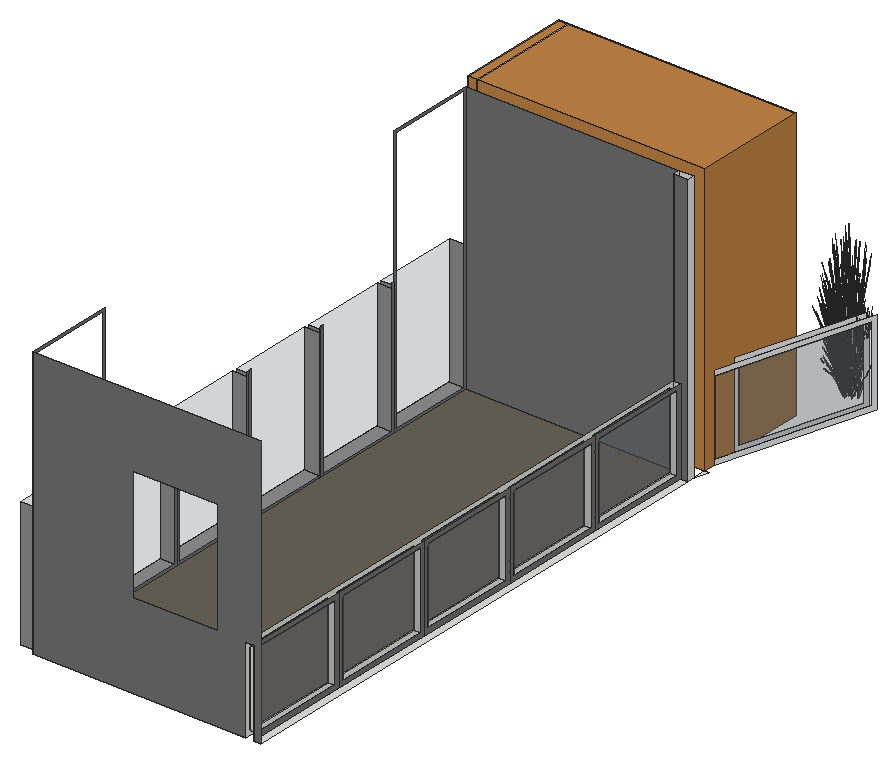
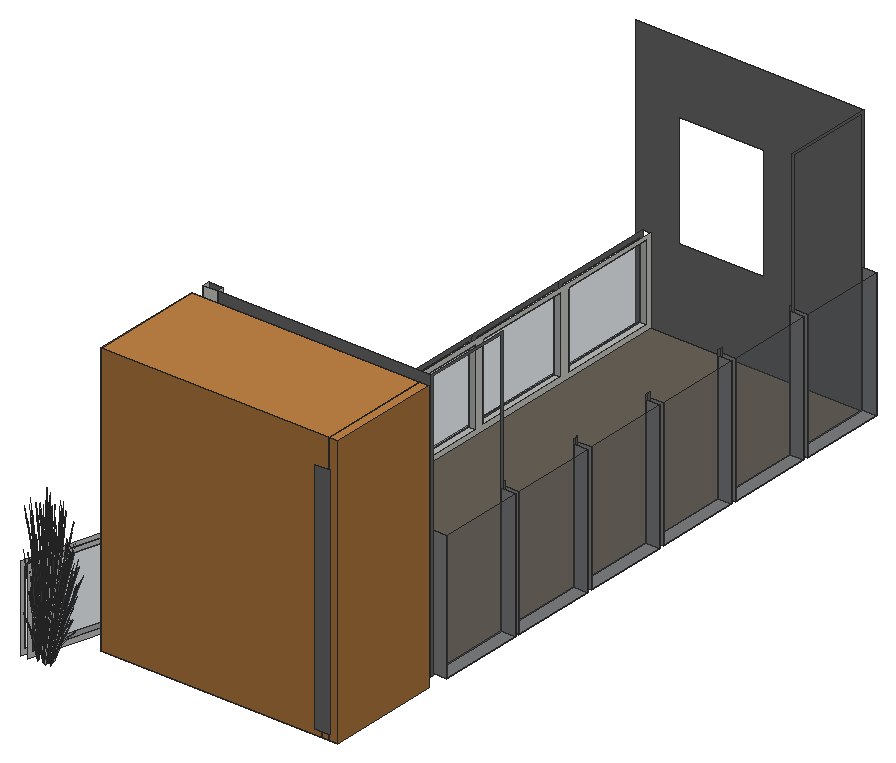
# SketchUp Ruby script. Lengths in inches.
U = 1.inch
M = Sketchup.active_model
def pt(a) = Geom::Point3d.new(a.map { |v| v * U })
def face(e, loops, mat)
  f = e.add_face(loops[0].map { |a| pt(a) })
  loops[1..].each { |l| e.add_face(l.map { |a| pt(a) }).erase! }
  f.material = f.back_material = mat if mat
  f
end
# faces: each face lists its corners as indices into pts; further lists are holes
def faces(e, pts, list, mat = nil) = list.each { |f| face(e, (f[0].is_a?(Array) ? f : [f]).map { |l| l.map { |i| pts[i] } }, mat) }
# xy, xz, yz: faces in a plane at the given z, y or x. An outline is a flat list of corners, or four numbers for a rectangle; further outlines are holes
def ring(l) = l.size == 4 ? [[l[0], l[1]], [l[2], l[1]], [l[2], l[3]], [l[0], l[3]]] : l.each_slice(2).to_a
def flat(e, list, mat, &to3) = list.each { |f| face(e, (f[0].is_a?(Array) ? f : [f]).map { |l| ring(l).map { |u, v| to3.(u, v) } }, mat) }
def xy(e, z, list, mat = nil) = flat(e, list, mat) { |x, y| [x, y, z] }
def xz(e, y, list, mat = nil) = flat(e, list, mat) { |x, z| [x, y, z] }
def yz(e, x, list, mat = nil) = flat(e, list, mat) { |y, z| [x, y, z] }
def lines(e, pts, list) = list.each { |a, b| e.add_line(pt(pts[a]), pt(pts[b])) }
# prism: a flat outline (further loops are holes) pulled along v
def prism(e, loops, v, mat = nil)
  f = face(e, loops, mat); d = Geom::Vector3d.new(v.map { |x| x * U })
  f.pushpull(f.normal.samedirection?(d) ? d.length : -d.length)
end
def box(e, o, s, mat = nil) = prism(e, [[o, [o[0] + s[0], o[1], o[2]], [o[0] + s[0], o[1] + s[1], o[2]], [o[0], o[1] + s[1], o[2]]]], [0, 0, s[2]], mat)
def at(x, y, z, deg = 0) = Geom::Transformation.translation(pt([x, y, z])) * Geom::Transformation.rotation(ORIGIN, Z_AXIS, deg.degrees)
def axes(o, x, y, z) = Geom::Transformation.new([*x, 0, *y, 0, *z, 0, *pt(o).to_a, 1])
def part(name) = M.definitions.add(name)
# library, detail: a bought-in or finely detailed component or shape, given as its bounding box
def library(name, o, s) = part(name).tap { |d| box(d.entities, o, s) }
def detail(e, o, s) = box(e.add_group.entities, o, s)
def put(e, d, t, mat = nil) = e.add_instance(d, t).tap { |i| i.material = mat if mat }
def group(e, t, mat = nil) = e.add_group.tap { |g| g.transformation = t; g.material = mat if mat }.entities
root = M.entities
M.materials.add("Glass_Basic_01").color = [105, 113, 122]
M.materials["Glass_Basic_01"].alpha = 0.25
M.materials.add("LightPink_Translucent").color = [144, 107, 117]
M.materials["LightPink_Translucent"].alpha = 0.75
M.materials.add("M01_Silver_Fog").color = [224, 224, 224]
M.materials.add("M04_Stone_Frost").color = [142, 142, 142]
M.materials.add("M06_Steel_Smoke").color = [114, 114, 114]
M.materials.add("Plaster_04_1K").color = [106, 98, 87]
M.materials.add("Wood_Floor_01_1K").color = [193, 132, 69]
c1 = part("Group\#1")
box(c1.entities,[-3.94,0,0],[99.94,48,114])
c2 = part("blade")
p = [[2.15,0.21,22],[0,0.17,0],[0.09,0.45,0],[2.18,0.31,22],[2.29,0.31,22],[0.38,0.45,0],
  [2.48,0.24,33],[2.49,0.24,33],[2.48,0.22,33]]
faces(c2.entities,p,[[0,1,2,3],[4,5,2,3],[6,3,4,7],[8,0,3,6]])
c3 = part("seeds")
p = [[0.3,-0.1,1.38],[-0.01,-0.03,1.59],[-0.01,-0.03,0.03],[0.14,-0.07,-0.07],[0.29,-0.03,3],[0.15,0.01,3.11]]
faces(c3.entities,p,[[0,1,2,3],[1,0,4,5]],"LightPink_Translucent")
c4 = part("blade with seeds")
put(c4.entities,c2,at(0,0,0))
put(c4.entities,c3,axes([2.4,0.25,30.99],[1.5799,-0.05474,1.17369],[-0.12525,1.92788,0.29478],[-0.07173,-0.02425,1.56792]))
xy(root,270,[[303,6,306,231],[306,234,307.76,240,306,240]])
xy(root,270,[[210,6,300,234]],"Plaster_04_1K")
xy(root,271,[[204,7,210,43],[204,45,210,81],[204,83,210,119],[204,121,210,157],[204,159,210,195],
  [204,197,210,233]],"M04_Stone_Frost")
xy(root,272,[[300,8,303,49],[300,53,303,94],[300,98,303,139],[300,143,303,184],[300,188,303,229]])
xz(root,6,[[[210,270,210,384,306,384,306,270,303,270,303,306,300,306,300,270],[252,306,288,354]]],"M06_Steel_Smoke")
xz(root,7,[[204,271,210,325]],"M04_Stone_Frost")
xz(root,8,[[300,272,303,304]])
xz(root,43,[[204,271,210,325]],"M04_Stone_Frost")
xz(root,45,[[204,271,210,325]],"M04_Stone_Frost")
xz(root,49,[[300,272,303,304]])
xz(root,53,[[300,272,303,304]])
xz(root,81,[[204,271,210,325]],"M04_Stone_Frost")
xz(root,83,[[204,271,210,325]],"M04_Stone_Frost")
xz(root,94,[[300,272,303,304]])
xz(root,98,[[300,272,303,304]])
xz(root,119,[[204,271,210,325]],"M04_Stone_Frost")
xz(root,121,[[204,271,210,325]],"M04_Stone_Frost")
xz(root,139,[[300,272,303,304]])
xz(root,143,[[300,272,303,304]])
xz(root,157,[[204,271,210,325]],"M04_Stone_Frost")
xz(root,159,[[204,271,210,325]],"M04_Stone_Frost")
xz(root,184,[[300,272,303,304]])
xz(root,188,[[300,272,303,304]])
xz(root,195,[[204,271,210,325]],"M04_Stone_Frost")
xz(root,197,[[204,271,210,325]],"M04_Stone_Frost")
xz(root,229,[[300,272,303,304]])
xz(root,231,[[303,270,306,270,306,384,300,384,300,306,303,306]],"M06_Steel_Smoke")
xz(root,233,[[204,271,210,325]],"M04_Stone_Frost")
xz(root,234,[[300,270,306,384]])
xz(root,234,[[210,270,300,384]],"M06_Steel_Smoke")
xz(root,243,[[213,270,305.51,306]],"M01_Silver_Fog")
xz(root,246,[[216,270,303.26,306]],"M01_Silver_Fog")
xz(root,287.79,[[213,270,216,306]],"M01_Silver_Fog")
xz(root,295,[[204,277,210,377]],"M06_Steel_Smoke")
yz(root,204,[[7,271,43,325],[45,271,81,325],[83,271,119,325],[121,271,157,325],[159,271,195,325],
  [197,271,233,325]],"Glass_Basic_01")
yz(root,210,[[240,270,288,270,288,316.46,286.46,316.46,286.46,337.54,288,337.54,288,384,240,384]])
yz(root,210,[[6,270,44,270,44,327,43,327,43,271,7,271,7,383,43,383,43,327,44,327,44,384,6,384],[44,270,82,270,82,327,81,327,81,271,45,271,45,327,44,327],[82,270,120,270,120,327,119,327,119,271,83,271,83,327,82,327],[120,270,158,270,158,327,157,327,157,271,121,271,121,327,120,327],[158,270,196,270,196,327,195,327,195,271,159,271,159,327,158,327],
  [196,270,234,270,234,384,196,384,196,327,197,327,197,383,233,383,233,271,197,271,197,327,196,327]],"M06_Steel_Smoke")
yz(root,213,[[243,270,287.79,306]],"M01_Silver_Fog")
yz(root,216,[[246,270,287.79,306]],"M01_Silver_Fog")
yz(root,300,[[[6,270,231,306],[8,272,49,304],[143,272,184,304],[188,272,229,304],[53,272,94,304],[98,272,139,304]],[231,270,234,384]])
yz(root,300,[[8,272,49,304],[53,272,94,304],[98,272,139,304],[143,272,184,304],[188,272,229,304]],"Glass_Basic_01")
yz(root,303,[[8,272,49,304],[53,272,94,304],[98,272,139,304],[143,272,184,304],[188,272,229,304]],"Glass_Basic_01")
yz(root,303,[[[6,270,51,306],[8,272,49,304]],[[51,270,96,306],[53,272,94,304]],[[96,270,141,306],[98,272,139,304]],[[141,270,186,306],[143,272,184,304]],[[186,270,231,306],[188,272,229,304]]],"M06_Steel_Smoke")
yz(root,306,[[231,270,234,384]])
p = [[305.51,243,270],[324.34,307.35,270],[324.34,307.35,306],[305.51,243,306],[323.78,305.43,304],[323.78,305.43,272],
  [306.07,244.92,272],[306.07,244.92,304],[303.26,246,306],[306,255.36,306],[306,255.36,270],[303.26,246,270],
  [321.22,307.35,306],[321.22,307.35,270],[320.65,305.43,304],[306.5625,257.28,304],[306.5625,257.28,272],[320.65,305.43,272],
  [209.78,288,384],[209.78,288,270],[305.48,242.91,270],[305.48,242.91,306]]
faces(root,p,[[[0,1,2,3],[4,5,6,7]],[8,9,10,11],[[9,12,13,10],[14,15,16,17]]],"M01_Silver_Fog")
faces(root,p,[[5,4,7,6],[15,14,17,16]],"Glass_Basic_01")
lines(root,p,[[18,19],[20,21]])
put(root,c1,at(210,240,270),"Wood_Floor_01_1K")
put(root,c4,axes([312.0625,305.99,273.875],[0.11485,0.17291,1.71376],[-0.53072,0.14557,0.13857],[-0.11995,-0.27145,0.73262]))
put(root,c4,axes([312.9375,304.84,274.72],[-0.07685,-0.07551,1.74944],[-0.51287,0.04787,-0.27667],[-0.08185,-0.1806,0.14031]))
put(root,c4,axes([314.125,305.74,272.59],[-0.14282,0.10901,1.43002],[-0.42773,-0.19079,-0.30754],[0.07929,-0.23728,0.61141]))
put(root,c4,axes([313.48,306.12,274.98],[-0.23981,-0.43789,-0.71045],[0.49365,-0.24404,0.08574],[-0.05608,-0.21158,1.00501]))
put(root,c4,axes([311.92,305.53,272.59],[-0.03043,0.17617,1.43002],[-0.4448,0.14748,-0.30754],[-0.10397,-0.22771,0.61141]))
put(root,c4,axes([313.0625,305.15,271.49],[-0.08428,0.0194,1.76342],[-0.46606,-0.21841,-0.26939],[0.00782,-0.18218,0.30037]))
put(root,c4,axes([314.47,306.55,274.98],[0.01307,-0.49815,-0.71045],[0.55054,0.03346,0.08574],[0.0581,-0.21104,1.00501]))
put(root,c4,axes([315.24,305.77,274.72],[-0.00485,-0.10718,1.74944],[-0.40965,-0.30977,-0.27667],[0.06333,-0.18778,0.14031]))
put(root,c4,axes([313.52,305.75,274.53],[0.15148,-0.41415,-0.35414],[0.44193,0.12079,0.4572],[-0.04052,-0.16674,0.87481]))
put(root,c4,axes([313.85,306.29,273.875],[-0.09355,0.18511,1.71376],[-0.39247,-0.38307,0.13857],[0.17705,-0.23875,0.73262]))
put(root,c4,axes([315.13,305.38,274.71],[-0.05103,0.04113,1.77383],[-0.49994,-0.13878,-0.16761],[-0.0181,-0.17951,0.31391]))
put(root,c4,axes([313.3,306.03,274.68],[-0.49392,-0.135,-0.51099],[0.1693,-0.46287,-0.3958],[-0.04529,-0.18636,0.97773]))
put(root,c4,axes([313.6,304.87,272.77],[0.06446,0.31404,1.1486],[-0.35756,-0.17393,0.84392],[0.03848,-0.1608,0.25299]))
put(root,c4,axes([314.36,306.38,274.68],[-0.35968,-0.36185,-0.51099],[0.37996,-0.3169,-0.3958],[0.05473,-0.18385,0.97773]))
put(root,c4,axes([312.41,304.6,274.71],[-0.00937,0.06455,1.77383],[-0.46231,0.23427,-0.16761],[-0.13604,-0.11975,0.31391]))
put(root,c4,axes([312.31,305.74,275.09],[0.55971,-0.13842,0.53763],[0.09714,0.54299,0.4433],[-0.13164,-0.16003,1.11249]))
put(root,c4,axes([313.58,305.84,274.73],[0.4951,0.14079,0.48003],[-0.1693,0.46287,0.3958],[-0.02975,-0.18203,0.9933]))
put(root,c4,axes([313.72,306.01,275.03],[-0.49168,0.25073,-0.1216],[-0.24162,-0.44501,-0.67495],[-0.06487,-0.18753,1.02557]))
put(root,c4,axes([314.74,306.57,275.03],[-0.55221,-0.02668,-0.1216],[0.01509,-0.50521,-0.67495],[0.03836,-0.19458,1.02557]))
put(root,c4,axes([314.7,306.25,274.53],[0.33997,-0.28354,-0.35414],[0.32182,0.32376,0.4572],[0.04897,-0.1645,0.87481]))
put(root,c4,axes([311.76,305.25,272.77],[0.2621,0.18744,1.1486],[-0.38171,0.11267,0.84392],[-0.08167,-0.14405,0.25299]))
put(root,c4,axes([313.71,305.81,274.73],[0.37023,-0.18303,0.0643],[0.18122,0.33376,0.50621],[-0.03575,-0.14712,0.77189]))
put(root,c4,axes([312.4,306.24,274.98],[-0.42844,-0.2603,-0.71045],[0.30448,-0.45614,0.08574],[-0.15523,-0.15542,1.00501]))
put(root,c4,axes([312.25,305.9,274.53],[-0.0776,-0.43378,-0.35414],[0.44361,-0.11454,0.4572],[-0.11915,-0.12431,0.87481]))
put(root,c4,axes([312.4375,305.86,274.73],[0.22836,-0.34211,0.0643],[0.3252,0.19918,0.50621],[-0.10513,-0.10968,0.77189]))
put(root,c4,axes([311.56,305.81,271.49],[-0.04867,0.07094,1.76342],[-0.49185,0.15296,-0.26939],[-0.11882,-0.13915,0.30037]))
put(root,c4,axes([312.37,307.76,272.1],[-0.20635,-0.55225,-0.69835],[0.59439,-0.19889,-0.18329],[-0.02281,-0.18701,1.54149]))
put(root,c4,axes([311.29,306.53,273.875],[0.18664,0.09279,1.71376],[-0.38624,0.38925,0.13857],[-0.24072,-0.1756,0.73262]))
put(root,c4,axes([315.125,306.08,271.49],[-0.0752,-0.04243,1.76342],[-0.19317,-0.47398,-0.26939],[0.13031,-0.12863,0.30037]))
put(root,c4,axes([313.57,306.18,275.05],[-0.15148,0.41415,0.35414],[-0.44193,-0.12079,-0.4572],[-0.04052,-0.16674,0.87481]))
put(root,c4,axes([312.19,306.26,274.68],[-0.4958,0.12802,-0.51099],[-0.08673,-0.48481,-0.3958],[-0.13317,-0.13893,0.97773]))
put(root,c4,axes([314.7,306.36,274.73],[0.35779,0.36745,0.48003],[-0.37996,0.3169,0.3958],[0.066,-0.17239,0.9933]))
put(root,c4,axes([312.54,305.82,275.43],[-0.33533,0.51628,-0.13619],[-0.48563,-0.29744,-0.75594],[-0.16881,-0.14586,1.14864]))
put(root,c4,axes([314.83,306.39,274.73],[0.4129,0.02509,0.0643],[-0.01132,0.37891,0.50621],[0.04321,-0.14514,0.77189]))
put(root,c4,axes([314.52,306.65,275.05],[-0.33997,0.28354,0.35414],[-0.32182,-0.32376,-0.4572],[0.04897,-0.1645,0.87481]))
put(root,c4,axes([315.12,307.41,274.98],[0.26246,-0.42493,-0.71045],[0.45991,0.30199,0.08574],[0.15671,-0.15395,1.00501]))
put(root,c4,axes([312.29,306.18,272.375],[-0.31414,-0.53965,0],[0.52557,-0.30095,-0.51607],[0.1197,-0.06854,1.63711]))
put(root,c4,axes([315.11,307.21,274.68],[-0.12908,-0.49174,-0.51099],[0.48882,-0.08602,-0.3958],[0.14008,-0.13208,0.97773]))
put(root,c4,axes([312.98,305.53,272.13],[-0.34721,0.30895,-0.03893],[-0.31814,-0.33837,-0.17649],[-0.0224,-0.09588,0.58215]))
put(root,c4,axes([311.26,305.67,274.72],[-0.10811,-0.0038,1.74944],[-0.34418,0.38014,-0.27667],[-0.18364,-0.07767,0.14031]))
put(root,c4,axes([315.34,307.57,275.03],[-0.46478,-0.29695,-0.1216],[0.26776,-0.43004,-0.67495],[0.13131,-0.14949,1.02557]))
put(root,c4,axes([313.42,309.1875,273.33],[0.4342,0.21716,1.51261],[-0.42537,0.46784,0.59816],[-0.19053,-0.27728,1.26806]))
put(root,c4,axes([312.51,306.25,275.05],[0.0776,0.43378,0.35414],[-0.44361,0.11454,-0.4572],[-0.11915,-0.12431,0.87481]))
put(root,c4,axes([311.15,307.6875,272.02],[0,-0.53854,-0.49651],[0.56215,0,0],[0,-0.12266,1.57504]))
put(root,c4,axes([312.71,306.09,272.02],[0.47024,-0.26927,-0.49651],[0.28107,0.48284,0],[0.1071,-0.06133,1.57504]))
put(root,c4,axes([315.5,307.02,272.59],[-0.1795,-0.01595,1.43002],[-0.18389,-0.42791,-0.30754],[0.22051,-0.12105,0.61141]))
put(root,c4,axes([311.18,306.53,275.09],[0.41494,-0.39744,0.53763],[0.35786,0.42207,0.4433],[-0.19468,-0.07331,1.11249]))
put(root,c4,axes([316.48,307.4375,274.71],[-0.06563,-0.00409,1.77383],[-0.27252,-0.43825,-0.16761],[0.10944,-0.1441,0.31391]))
put(root,c4,axes([313.27,307.2,272.06],[0.33843,-0.40479,-0.62353],[0.42041,0.36705,-0.16365],[0.13561,-0.10098,1.37633]))
put(root,c4,axes([315.71,306.24,272.77],[-0.16736,0.27414,1.1486],[-0.14385,-0.36832,0.84392],[0.13822,-0.09229,0.25299]))
put(root,c4,axes([315.47,307.27,274.53],[0.43736,-0.07697,-0.35414],[0.11549,0.43998,0.4572],[0.12533,-0.11818,0.87481]))
put(root,c4,axes([311.37,306.53,274.73],[0.0253,-0.40952,0.0643],[0.38204,0.01123,0.50621],[-0.14634,-0.04285,0.77189]))
put(root,c4,axes([312.68,307.91,272.21],[0.24378,-0.48527,-0.44739],[0.50654,0.23354,0.21531],[0,-0.11186,1.43643]))
put(root,c4,axes([311.22,306.66,274.53],[-0.28589,-0.33718,-0.35414],[0.32644,-0.31919,0.4572],[-0.16586,-0.04856,0.87481]))
put(root,c4,axes([312.9,307.67,272.67],[-0.05855,-0.61451,-0.29095],[0.60981,-0.03716,-0.50002],[0.10738,-0.08185,1.59708]))
put(root,c4,axes([311.39,307.7,272.03],[0.35073,-0.33601,-0.30978],[0.35073,0.33601,0.30978],[0,-0.10823,1.38974]))
put(root,c4,axes([311.25,306.09,272.13],[-0.14494,0.43975,-0.03893],[-0.4461,-0.13527,-0.17649],[-0.06773,-0.07192,0.58215]))
put(root,c4,axes([315.11,307.53,275.05],[-0.43736,0.07697,0.35414],[-0.11549,-0.43998,-0.4572],[0.12533,-0.11818,0.87481]))
put(root,c4,axes([312.62,308.31,272.67],[-0.56585,-0.25696,-0.29095],[0.27246,-0.54236,-0.50002],[-0.01778,-0.13316,1.59708]))
put(root,c4,axes([311.01,308.1,272.375],[-0.62828,0,0],[0,-0.6019,-0.51607],[0,-0.13709,1.63711]))
put(root,c4,axes([311.12,307.02,272.59],[0.0981,0.14994,1.43002],[-0.22605,0.40756,-0.30754],[-0.23211,-0.09741,0.61141]))
put(root,c4,axes([312.82,306.31,272.03],[0.46876,0.13325,-0.30978],[-0.11803,0.46926,0.30978],[0.0945,-0.05411,1.38974]))
put(root,c4,axes([311.52,306.89,274.98],[-0.50227,-0.01297,-0.71045],[0.03373,-0.54602,0.08574],[-0.21278,-0.05762,1.00501]))
put(root,c4,axes([315.51,307.46,274.73],[0.34493,0.22649,0.0643],[-0.20082,0.32253,0.50621],[0.11059,-0.10427,0.77189]))
put(root,c4,axes([315.41,307.36,274.73],[0.12461,0.49565,0.48003],[-0.48882,0.08602,0.3958],[0.14406,-0.11657,0.9933]))
put(root,c4,axes([316.73,307.96,274.72],[0.06972,-0.08203,1.74944],[-0.08924,-0.50318,-0.27667],[0.17494,-0.0954,0.14031]))
put(root,c4,axes([311.5,307.9375,272.33],[-0.46736,0.45277,0.30756],[-0.46764,-0.44801,-0.36492],[-0.01632,-0.12858,1.64885]))
put(root,c4,axes([310.84,306,274.71],[0.03725,0.05374,1.77383],[-0.17957,0.48312,-0.16761],[-0.18186,0.0035,0.31391]))
put(root,c4,axes([312.98,308.15,272.43],[0.56613,0.26102,0.24065],[-0.27246,0.54236,0.50002],[0,-0.12502,1.60543]))
put(root,c4,axes([312.76,308.88,272.4375],[0.13317,-0.63814,-0.23429],[0.63143,0.11124,0.51271],[-0.11033,-0.08813,1.5644]))
put(root,c4,axes([311.36,307,274.68],[-0.36484,0.35674,-0.51099],[-0.31952,-0.37685,-0.3958],[-0.18537,-0.05428,0.97773]))
put(root,c4,axes([311.625,306.84,275.05],[0.28589,0.33718,0.35414],[-0.32644,0.31919,-0.4572],[-0.16586,-0.04856,0.87481]))
put(root,c4,axes([310.53,307.47,272.77],[0.32078,-0.03854,1.1486],[-0.20348,0.33954,0.84392],[-0.15852,-0.05093,0.25299]))
put(root,c4,axes([312.8,307.78,272.72],[-0.54562,0.03324,0.44739],[-0.04934,-0.55185,-0.21531],[0.09768,-0.05593,1.43643]))
put(root,c4,axes([311.55,306.625,275.03],[-0.0269,0.54769,-0.1216],[-0.50939,-0.01497,-0.67495],[-0.19618,-0.03804,1.02557]))
put(root,c4,axes([311.39,308.1875,272.48],[0,0.53854,0.49651],[-0.56215,0,0],[0,-0.12266,1.57504]))
put(root,c4,axes([315.36,308.73,275.03],[-0.25281,-0.48765,-0.1216],[0.44869,-0.23964,-0.67495],[0.18908,-0.06434,1.02557]))
put(root,c4,axes([315.34,308.31,274.68],[0.13612,-0.48987,-0.51099],[0.46669,0.16791,-0.3958],[0.1879,-0.04492,0.97773]))
put(root,c4,axes([314.6,306.3125,272.375],[0.31414,-0.53965,0],[0.52557,0.30095,-0.51607],[0.1197,0.06854,1.63711]))
put(root,c4,axes([310.9,307.38,273.875],[0.20841,-0.0122,1.71376],[-0.13825,0.52864,0.13857],[-0.297,-0.0327,0.73262]))
put(root,c4,axes([312.72,308.62,272.21],[-0.30184,-0.45202,-0.44739],[0.45719,-0.31831,0.21531],[-0.09768,-0.05593,1.43643]))
put(root,c4,axes([312.78,307.98,272.36],[0.21845,0.6022,0.45755],[-0.62418,0.20941,0.17955],[0.00763,-0.11065,1.58856]))
put(root,c4,axes([315.84,308.44,271.98],[-0.32361,0.06463,1.41583],[-0.05151,-0.51444,0.08104],[0.22666,-0.07786,0.80566]))
put(root,c4,axes([316.42,307.99,272.26],[-0.31151,-0.34437,-0.06488],[0.34117,-0.31553,-0.29416],[0.09667,-0.02221,0.97024]))
put(root,c4,axes([312.67,308.46,272.72],[-0.24378,0.48527,0.44739],[-0.50654,-0.23354,-0.21531],[0,-0.11186,1.43643]))
put(root,c4,axes([313.57,308.03,272.21],[0,-0.62313,0],[0.62828,0,0],[0,0,1.79456]))
put(root,c4,axes([314.33,306.59,272.48],[-0.47024,-0.26927,0.49651],[0.28107,-0.48284,0],[0.1071,0.06133,1.57504]))
put(root,c4,axes([315.25,308.49,274.98],[0.44151,-0.23785,-0.71045],[0.24605,0.4896,0.08574],[0.21333,-0.05562,1.00501]))
put(root,c4,axes([312.45,308.79,272.06],[-0.52267,-0.08829,-0.62353],[0.11029,-0.54463,-0.16365],[-0.15598,-0.06599,1.37633]))
put(root,c4,axes([313.27,307.64,272.36],[-0.4166,0.48873,0.45755],[-0.49494,-0.43142,0.17955],[0.10044,-0.04877,1.58856]))
put(root,c4,axes([313.72,308.52,272.3],[-0.46736,-0.46353,-0.06131],[0.46764,-0.46381,0],[-0.01632,-0.01619,1.75571]))
put(root,c4,axes([312.55,306.84,272.47],[-0.14515,0.53522,0.17642],[-0.53115,-0.15146,0.35086],[0.09175,-0.00261,1.60407]))
put(root,c4,axes([315.18,308.58,275.05],[-0.41757,-0.15024,0.35414],[0.12179,-0.4383,-0.4572],[0.16812,-0.04019,0.87481]))
put(root,c4,axes([310.8125,307.78,274.73],[0.14195,-0.49104,0.48003],[0.46669,0.16791,0.3958],[-0.18353,0.02951,0.9933]))
put(root,c4,axes([312.33,307.27,271.59],[-0.49456,0.21561,1.28929],[-0.15741,-0.61865,0.50096],[0.30369,0.01029,1.46642]))
put(root,c4,axes([313.65,307.43,272.62],[0.09693,-0.48062,0.1448],[0.47357,0.08343,-0.41347],[0.08619,0.04935,1.26744]))
put(root,c4,axes([310.78,307.65,274.73],[-0.18454,-0.3672,0.0643],[0.33652,-0.17973,0.50621],[-0.14834,0.03546,0.77189]))
put(root,c4,axes([312.84,308.57,272.36],[0.63506,0.11347,0.45755],[-0.12924,0.64083,0.17955],[-0.09281,-0.06188,1.58856]))
put(root,c4,axes([316.1875,308.11,271.49],[-0.02626,-0.08176,1.76342],[0.18213,-0.47826,-0.26939],[0.18372,-0.00688,0.30037]))
put(root,c4,axes([310.77,308.03,271.49],[0.01274,0.08487,1.76342],[-0.25688,0.44323,-0.26939],[-0.18246,-0.02234,0.30037]))
put(root,c4,axes([313.45,307.56,272.72],[-0.30184,-0.45202,0.44739],[0.45719,-0.31831,-0.21531],[0.09768,0.05593,1.43643]))
put(root,c4,axes([311.89,309.625,272.03],[-0.11803,-0.46926,-0.30978],[0.46876,-0.13325,0.30978],[-0.0945,-0.05411,1.38974]))
put(root,c4,axes([312.49,309.6,272.47],[0.53992,-0.14294,0.17642],[0.13332,0.53195,0.35086],[-0.04815,-0.07751,1.60407]))
put(root,c4,axes([313.61,307.59,272.67],[0.5073,-0.35754,-0.29095],[0.33735,0.5052,-0.50002],[0.12516,0.05131,1.59708]))
